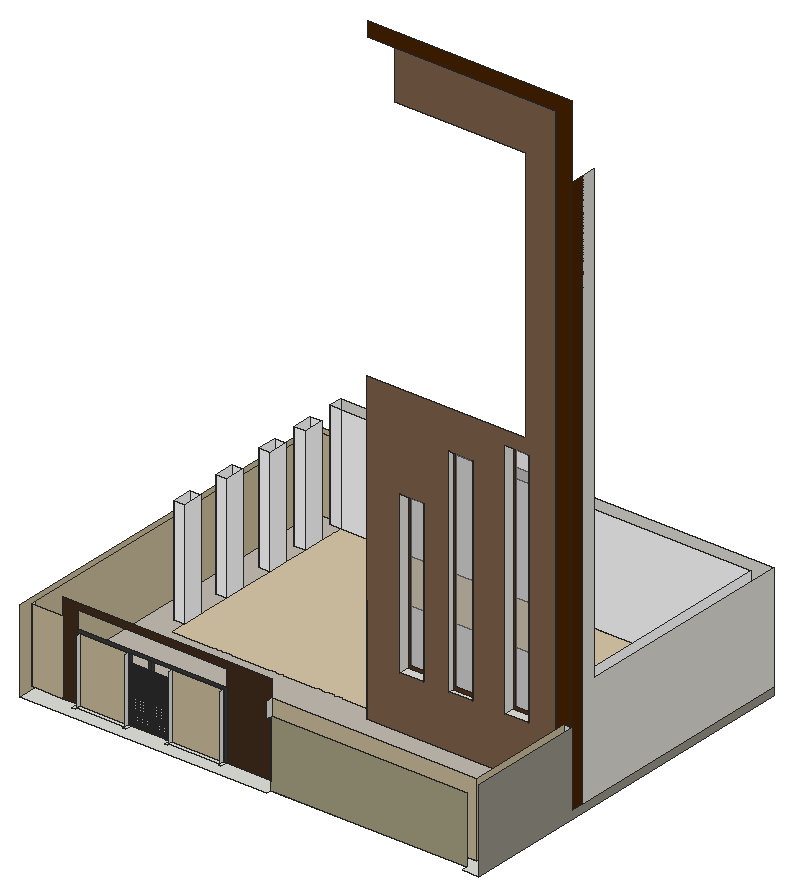
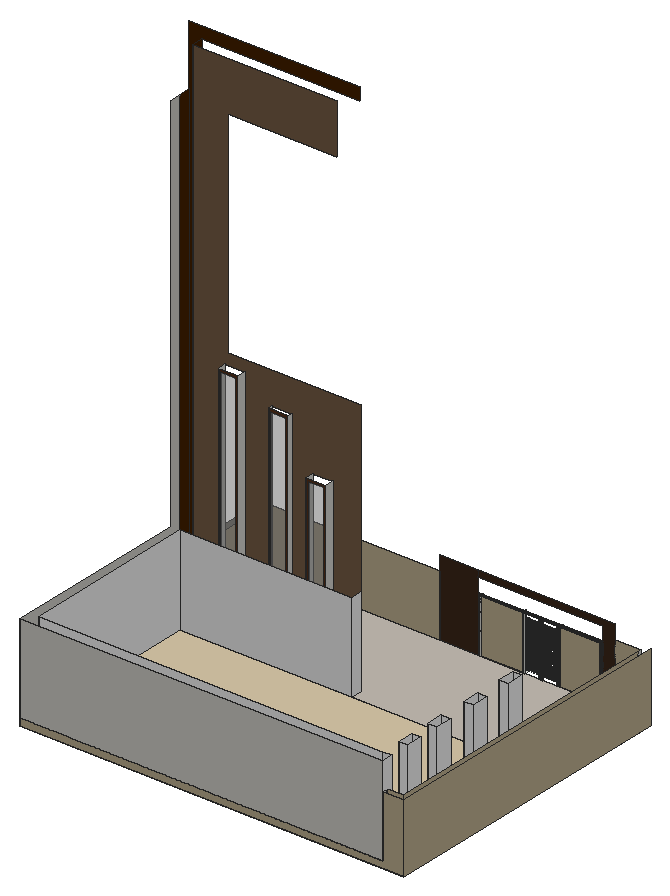
# SketchUp Ruby script. Lengths in inches.
U = 1.inch
M = Sketchup.active_model
def pt(a) = Geom::Point3d.new(a.map { |v| v * U })
def face(e, loops, mat)
  f = e.add_face(loops[0].map { |a| pt(a) })
  loops[1..].each { |l| e.add_face(l.map { |a| pt(a) }).erase! }
  f.material = f.back_material = mat if mat
  f
end
# faces: each face lists its corners as indices into pts; further lists are holes
def faces(e, pts, list, mat = nil) = list.each { |f| face(e, (f[0].is_a?(Array) ? f : [f]).map { |l| l.map { |i| pts[i] } }, mat) }
# xy, xz, yz: faces in a plane at the given z, y or x. An outline is a flat list of corners, or four numbers for a rectangle; further outlines are holes
def ring(l) = l.size == 4 ? [[l[0], l[1]], [l[2], l[1]], [l[2], l[3]], [l[0], l[3]]] : l.each_slice(2).to_a
def flat(e, list, mat, &to3) = list.each { |f| face(e, (f[0].is_a?(Array) ? f : [f]).map { |l| ring(l).map { |u, v| to3.(u, v) } }, mat) }
def xy(e, z, list, mat = nil) = flat(e, list, mat) { |x, y| [x, y, z] }
def xz(e, y, list, mat = nil) = flat(e, list, mat) { |x, z| [x, y, z] }
def yz(e, x, list, mat = nil) = flat(e, list, mat) { |y, z| [x, y, z] }
def lines(e, pts, list) = list.each { |a, b| e.add_line(pt(pts[a]), pt(pts[b])) }
# prism: a flat outline (further loops are holes) pulled along v
def prism(e, loops, v, mat = nil)
  f = face(e, loops, mat); d = Geom::Vector3d.new(v.map { |x| x * U })
  f.pushpull(f.normal.samedirection?(d) ? d.length : -d.length)
end
def box(e, o, s, mat = nil) = prism(e, [[o, [o[0] + s[0], o[1], o[2]], [o[0] + s[0], o[1] + s[1], o[2]], [o[0], o[1] + s[1], o[2]]]], [0, 0, s[2]], mat)
def at(x, y, z, deg = 0) = Geom::Transformation.translation(pt([x, y, z])) * Geom::Transformation.rotation(ORIGIN, Z_AXIS, deg.degrees)
def axes(o, x, y, z) = Geom::Transformation.new([*x, 0, *y, 0, *z, 0, *pt(o).to_a, 1])
def part(name) = M.definitions.add(name)
# library, detail: a bought-in or finely detailed component or shape, given as its bounding box
def library(name, o, s) = part(name).tap { |d| box(d.entities, o, s) }
def detail(e, o, s) = box(e.add_group.entities, o, s)
def put(e, d, t, mat = nil) = e.add_instance(d, t).tap { |i| i.material = mat if mat }
def group(e, t, mat = nil) = e.add_group.tap { |g| g.transformation = t; g.material = mat if mat }.entities
root = M.entities
M.materials.add("[Carrera Marble]").color = [252, 252, 252]
M.materials.add("[Carrera Marble]1").color = [247, 247, 247]
M.materials.add("[Cladding Siding Tan]").color = [124, 97, 73]
M.materials.add("[Color C08]").color = [71, 35, 0]
M.materials.add("[Color M07]").color = [58, 58, 58]
M.materials.add("[Field Rectangle Tile]").color = [196, 189, 179]
M.materials.add("[Field Square Tile]").color = [217, 201, 169]
M.materials.add("[Formica Graystone]1").color = [149, 146, 135]
M.materials.add("[Formica Speckled Grey]").color = [94, 105, 111]
M.materials.add("[Quartz Light Brown]").color = [199, 184, 152]
M.materials.add("[Sandstone]").color = [63, 43, 28]
M.materials.add("[Stone Coursed Rough]").color = [165, 160, 130]
M.materials.add("[Terrazzo Tile Light]").color = [219, 217, 210]
M.materials.add("[Translucent Glass Gray]1").color = [163, 163, 163]
M.materials["[Translucent Glass Gray]1"].alpha = 0.5
M.materials.add("[Wood Cherry Original]").color = [91, 51, 25]
xy(root,0,[[71.32,279.21,71.32,742.77,649.65,742.77,649.65,279.21,628.99,279.21,628.99,285.9,381.67,285.9,381.67,279.21]])
xy(root,10.08,[[136.3,279.21,140.74,288.34],[201.14,279.21,204.61,288.34],[253.76,279.21,256.89,288.34],[321.11,279.21,324.42,288.34],[140.74,281.7,201.14,286.88],
  [256.89,281.7,321.11,286.72],[256.89,286.72,321.11,288.34],[630.01,424.96,630.01,442.77,635.51,460.01,635.51,725.53,104.01,725.53,104.01,742.77,649.65,742.77,649.65,424.96],[376.83,442.77,376.83,460.01,635.51,460.01,630.01,442.77],[104.01,479.96,118.15,505.27],
  [104.01,546.4,118.15,571.71],[104.01,614.47,118.15,639.78],[104.01,670,118.15,695.31]])
xy(root,10.08,[[140.74,286.88,201.14,288.34]],"[Color M07]")
xy(root,10.08,[[78.57,288.34,639.83,288.34,639.83,424.96,630.01,424.96,630.01,442.77,376.83,442.77,376.83,460.01,118.15,460.01,118.15,479.96,104.01,479.96,104.01,505.27,118.15,505.27,118.15,546.4,104.01,546.4,104.01,571.71,118.15,571.71,118.15,614.47,104.01,614.47,104.01,639.78,118.15,639.78,118.15,670,104.01,670,104.01,695.31,118.15,695.31,118.15,725.53,104.01,725.53,104.01,734.15,78.57,734.15]],"[Field Rectangle Tile]")
xy(root,10.08,[[118.15,460.01,635.51,725.53]],"[Field Square Tile]")
xy(root,76.96,[[419.27,442.77,449.02,455.21],[480.71,442.77,510.46,449.52],[551.08,442.77,580.83,455.77]])
xz(root,285.9,[[381.67,0,628.99,83.9375]],"[Stone Coursed Rough]")
xz(root,286.72,[[256.89,10.08,321.11,91.34]],"[Quartz Light Brown]")
xz(root,286.88,[[140.74,10.08,201.14,91.34]],"[Quartz Light Brown]")
xz(root,288.34,[[253.76,10.08,256.89,91.34]])
xz(root,288.34,[[136.3,10.08,136.3,94.91,319.42,94.91,319.42,91.34,140.74,91.34,140.74,10.08],[201.14,10.08,204.61,91.34],[225.67,10.08,229.25,91.34],[229.25,10.08,232.82,91.34],[321.11,10.08,321.11,91.34,319.42,91.34,319.42,94.91,324.42,94.91,324.42,10.08]],"[Color M07]")
xz(root,288.34,[[78.57,10.08,118.15,103.14],[381.67,10.08,639.83,103.14]],"[Quartz Light Brown]")
xz(root,288.34,[[118.15,10.08,118.15,124.77,324.42,124.77,324.42,116.23,136.3,116.23,136.3,10.08],[324.42,10.08,381.67,124.77]],"[Sandstone]")
xz(root,424.96,[[639.83,10.08,649.65,103.14]])
xz(root,424.96,[[630.01,10.08,639.83,10.08,639.83,103.14,649.65,103.14,649.65,812.1,392.48,812.1,392.48,793.89,630.01,793.89]],"[Color C08]")
xz(root,442.77,[[[376.83,10.08,630.01,10.08,630.01,793.89,412.79,793.89,412.79,719.42,577.15,719.42,577.15,397.48,376.83,397.48],[551.08,76.96,580.83,380.34],[480.71,76.96,510.46,348.79],[419.27,76.96,449.02,278.96]]],"[Cladding Siding Tan]")
xz(root,449.52,[[484.53,80.79,506.63,344.96]],"[Translucent Glass Gray]1")
xz(root,449.52,[[[480.71,76.96,510.46,348.79],[484.53,80.79,506.63,344.96]]],"[Wood Cherry Original]")
xz(root,455.21,[[423.09,80.79,445.19,275.13]],"[Translucent Glass Gray]1")
xz(root,455.21,[[[419.27,76.96,449.02,278.96],[423.09,80.79,445.19,275.13]]],"[Wood Cherry Original]")
xz(root,455.77,[[554.91,80.79,577,376.52]],"[Translucent Glass Gray]1")
xz(root,455.77,[[[551.08,76.96,580.83,380.34],[554.91,80.79,577,376.52]]],"[Wood Cherry Original]")
xz(root,460.01,[[376.83,10.08,635.51,144.48]],"[Carrera Marble]1")
xz(root,479.96,[[104.01,10.08,118.15,144.48]],"[Carrera Marble]")
xz(root,505.27,[[104.01,10.08,118.15,144.48]],"[Carrera Marble]")
xz(root,546.4,[[104.01,10.08,118.15,144.48]],"[Carrera Marble]")
xz(root,571.71,[[104.01,10.08,118.15,144.48]],"[Carrera Marble]")
xz(root,614.47,[[104.01,10.08,118.15,144.48]],"[Carrera Marble]")
xz(root,639.78,[[104.01,10.08,118.15,144.48]],"[Carrera Marble]")
xz(root,670,[[104.01,10.08,118.15,144.48]],"[Carrera Marble]")
xz(root,695.31,[[104.01,10.08,118.15,144.48]],"[Carrera Marble]")
xz(root,725.53,[[118.15,10.08,635.51,144.48]],"[Carrera Marble]")
xz(root,725.53,[[104.01,10.08,118.15,144.48]],"[Carrera Marble]1")
xz(root,734.15,[[78.57,10.08,104.01,103.14]],"[Quartz Light Brown]")
xz(root,742.77,[[71.32,0,71.32,103.14,104.01,103.14,104.01,10.08,649.65,10.08,649.65,0]],"[Quartz Light Brown]")
xz(root,742.77,[[104.01,10.08,649.65,144.48]],"[Terrazzo Tile Light]")
yz(root,71.32,[[279.21,0,742.77,103.14]],"[Quartz Light Brown]")
yz(root,78.57,[[288.34,10.08,293.84,103.14]])
yz(root,78.57,[[293.84,10.08,734.15,103.14]],"[Quartz Light Brown]")
yz(root,104.01,[[734.15,10.08,742.77,103.14]])
yz(root,104.01,[[479.96,10.08,505.27,144.48],[546.4,10.08,571.71,144.48],[614.47,10.08,639.78,144.48],[670,10.08,695.31,144.48],[725.53,10.08,725.53,144.48,742.77,144.48,742.77,103.14,734.15,103.14,734.15,10.08]],"[Carrera Marble]")
yz(root,118.15,[[479.96,10.08,505.27,144.48],[546.4,10.08,571.71,144.48],[614.47,10.08,639.78,144.48],[670,10.08,695.31,144.48]],"[Carrera Marble]")
yz(root,140.74,[[281.7,10.08,286.88,91.34]])
yz(root,140.74,[[286.88,10.08,288.34,91.34]],"[Color M07]")
yz(root,201.14,[[281.7,10.08,286.88,91.34],[286.88,10.08,288.34,91.34]])
yz(root,256.89,[[281.7,10.08,286.72,91.34]])
yz(root,256.89,[[286.72,10.08,288.34,91.34]],"[Color M07]")
yz(root,321.11,[[281.7,10.08,286.72,91.34],[286.72,10.08,288.34,91.34]])
yz(root,376.83,[[442.77,10.08,460.01,144.48]],"[Carrera Marble]")
yz(root,381.67,[[285.9,10.08,288.34,10.08,288.34,103.14,279.21,103.14,279.21,83.9375,285.9,83.9375]])
yz(root,419.27,[[442.77,76.96,455.21,278.96]])
yz(root,449.02,[[442.77,76.96,455.21,278.96]])
yz(root,480.71,[[442.77,76.96,449.52,348.79]])
yz(root,510.46,[[442.77,76.96,449.52,348.79]])
yz(root,551.08,[[442.77,76.96,455.77,380.34]])
yz(root,580.83,[[442.77,76.96,455.77,380.34]])
yz(root,630.01,[[424.96,10.08,442.77,793.89]],"[Color C08]")
yz(root,635.51,[[460.01,10.08,725.53,144.48]],"[Carrera Marble]")
yz(root,639.83,[[288.34,10.08,424.96,103.14]],"[Quartz Light Brown]")
yz(root,649.65,[[424.96,10.08,442.77,719.42]],"[Color C08]")
yz(root,649.65,[[279.21,0,742.77,0,742.77,10.08,424.96,10.08,424.96,103.14,279.21,103.14]],"[Formica Graystone]1")
yz(root,649.65,[[442.77,10.08,742.77,10.08,742.77,144.48,460.01,144.48,460.01,719.42,442.77,719.42]],"[Terrazzo Tile Light]")
p = [[204.61,283.9,12.47],[204.61,284.05,12.53],[253.76,284.05,12.53],[253.76,283.9,12.47],[204.61,284.18,12.63],[253.76,284.18,12.63],
  [204.61,284.28,12.76],[253.76,284.28,12.76],[204.61,284.34,12.91],[253.76,284.34,12.91],[204.61,284.37,13.07],[253.76,284.37,13.07],
  [204.61,284.34,13.23],[253.76,284.34,13.23],[204.61,284.28,13.38],[253.76,284.28,13.38],[204.61,284.18,13.51],[253.76,284.18,13.51],
  [204.61,284.05,13.61],[253.76,284.05,13.61],[204.61,283.9,13.68],[253.76,283.9,13.68],[204.61,283.9,15.78],[204.61,284.05,15.84],
  [253.76,284.05,15.84],[253.76,283.9,15.78],[204.61,284.18,15.94],[253.76,284.18,15.94],[204.61,284.28,16.07],[253.76,284.28,16.07],
  [204.61,284.34,16.22],[253.76,284.34,16.22],[204.61,284.37,16.38],[253.76,284.37,16.38],[204.61,284.34,16.55],[253.76,284.34,16.55],
  [204.61,284.28,16.7],[253.76,284.28,16.7],[204.61,284.18,16.83],[253.76,284.18,16.83],[204.61,284.05,16.93],[253.76,284.05,16.93],
  [204.61,283.9,16.99],[253.76,283.9,16.99],[204.61,283.9,19.09],[204.61,284.05,19.16],[253.76,284.05,19.16],[253.76,283.9,19.09],
  [204.61,284.18,19.25],[253.76,284.18,19.25],[204.61,284.28,19.38],[253.76,284.28,19.38],[204.61,284.34,19.54],[253.76,284.34,19.54],
  [204.61,284.37,19.7],[253.76,284.37,19.7],[204.61,284.34,19.86],[253.76,284.34,19.86],[204.61,284.28,20.01],[253.76,284.28,20.01],
  [204.61,284.18,20.14],[253.76,284.18,20.14],[204.61,284.05,20.24],[253.76,284.05,20.24],[204.61,283.9,20.3],[253.76,283.9,20.3],
  [204.61,283.9,22.41],[204.61,284.05,22.47],[253.76,284.05,22.47],[253.76,283.9,22.41],[204.61,284.18,22.57],[253.76,284.18,22.57],
  [204.61,284.28,22.7],[253.76,284.28,22.7],[204.61,284.34,22.85],[253.76,284.34,22.85],[204.61,284.37,23.01],[253.76,284.37,23.01],
  [204.61,284.34,23.17],[253.76,284.34,23.17],[204.61,284.28,23.32],[253.76,284.28,23.32],[204.61,284.18,23.45],[253.76,284.18,23.45],
  [204.61,284.05,23.55],[253.76,284.05,23.55],[204.61,283.9,23.61],[253.76,283.9,23.61],[204.61,283.9,25.72],[204.61,284.05,25.78],
  [253.76,284.05,25.78],[253.76,283.9,25.72],[204.61,284.18,25.88],[253.76,284.18,25.88],[204.61,284.28,26.01],[253.76,284.28,26.01],
  [204.61,284.34,26.16],[253.76,284.34,26.16],[204.61,284.37,26.32],[253.76,284.37,26.32],[204.61,284.34,26.48],[253.76,284.34,26.48],
  [204.61,284.28,26.63],[253.76,284.28,26.63],[204.61,284.18,26.76],[253.76,284.18,26.76],[204.61,284.05,26.86],[253.76,284.05,26.86],
  [204.61,283.9,26.93],[253.76,283.9,26.93],[204.61,283.9,29.03],[204.61,284.05,29.09],[253.76,284.05,29.09],[253.76,283.9,29.03],
  [204.61,284.18,29.19],[253.76,284.18,29.19],[204.61,284.28,29.32],[253.76,284.28,29.32],[204.61,284.34,29.47],[253.76,284.34,29.47],
  [204.61,284.37,29.63],[253.76,284.37,29.63],[204.61,284.34,29.8],[253.76,284.34,29.8],[204.61,284.28,29.95],[253.76,284.28,29.95],
  [204.61,284.18,30.08],[253.76,284.18,30.08],[204.61,284.05,30.18],[253.76,284.05,30.18],[204.61,283.9,30.24],[253.76,283.9,30.24],
  [204.61,283.74,32.32],[204.61,283.9,32.34],[253.76,283.9,32.34],[253.76,283.74,32.32],[204.61,284.05,32.41],[253.76,284.05,32.41],
  [204.61,284.18,32.5],[253.76,284.18,32.5],[204.61,284.28,32.63],[253.76,284.28,32.63],[204.61,284.34,32.79],[253.76,284.34,32.79],
  [204.61,284.37,32.95],[253.76,284.37,32.95],[204.61,284.34,33.11],[253.76,284.34,33.11],[204.61,284.28,33.26],[253.76,284.28,33.26],
  [204.61,284.18,33.39],[253.76,284.18,33.39],[204.61,284.05,33.49],[253.76,284.05,33.49],[204.61,283.9,33.55],[253.76,283.9,33.55],
  [204.61,283.74,33.57],[253.76,283.74,33.57],[204.61,283.74,35.63],[204.61,283.9,35.66],[253.76,283.9,35.66],[253.76,283.74,35.63],
  [204.61,284.05,35.72],[253.76,284.05,35.72],[204.61,284.18,35.82],[253.76,284.18,35.82],[204.61,284.28,35.95],[253.76,284.28,35.95],
  [204.61,284.34,36.1],[253.76,284.34,36.1],[204.61,284.37,36.26],[253.76,284.37,36.26],[204.61,284.34,36.42],[253.76,284.34,36.42],
  [204.61,284.28,36.57],[253.76,284.28,36.57],[204.61,284.18,36.7],[253.76,284.18,36.7],[204.61,284.05,36.8],[253.76,284.05,36.8],
  [204.61,283.9,36.86],[253.76,283.9,36.86],[204.61,283.74,36.88],[253.76,283.74,36.88],[204.61,283.74,38.95],[204.61,283.9,38.97],
  [253.76,283.9,38.97],[253.76,283.74,38.95],[204.61,284.05,39.03],[253.76,284.05,39.03],[204.61,284.18,39.13],[253.76,284.18,39.13],
  [204.61,284.28,39.26],[253.76,284.28,39.26],[204.61,284.34,39.41],[253.76,284.34,39.41],[204.61,284.37,39.57],[253.76,284.37,39.57],
  [204.61,284.34,39.73],[253.76,284.34,39.73],[204.61,284.28,39.88],[253.76,284.28,39.88],[204.61,284.18,40.01],[253.76,284.18,40.01],
  [204.61,284.05,40.11],[253.76,284.05,40.11],[204.61,283.9,40.18],[253.76,283.9,40.18],[204.61,283.74,40.2],[253.76,283.74,40.2],
  [204.61,283.74,42.26],[204.61,283.9,42.28],[253.76,283.9,42.28],[253.76,283.74,42.26],[204.61,284.05,42.34],[253.76,284.05,42.34],
  [204.61,284.18,42.44],[253.76,284.18,42.44],[204.61,284.28,42.57],[253.76,284.28,42.57],[204.61,284.34,42.72],[253.76,284.34,42.72],
  [204.61,284.37,42.88],[253.76,284.37,42.88],[204.61,284.34,43.05],[253.76,284.34,43.05],[204.61,284.28,43.2],[253.76,284.28,43.2],
  [204.61,284.18,43.33],[253.76,284.18,43.33],[204.61,284.05,43.43],[253.76,284.05,43.43],[204.61,283.9,43.49],[253.76,283.9,43.49],
  [204.61,283.74,43.51],[253.76,283.74,43.51],[204.61,283.74,45.57],[204.61,283.9,45.59],[253.76,283.9,45.59],[253.76,283.74,45.57],
  [204.61,284.05,45.66],[253.76,284.05,45.66],[204.61,284.18,45.75],[253.76,284.18,45.75],[204.61,284.28,45.88],[253.76,284.28,45.88],
  [204.61,284.34,46.04],[253.76,284.34,46.04],[204.61,284.37,46.2],[253.76,284.37,46.2],[204.61,284.34,46.36],[253.76,284.34,46.36],
  [204.61,284.28,46.51],[253.76,284.28,46.51],[204.61,284.18,46.64],[253.76,284.18,46.64],[204.61,284.05,46.74],[253.76,284.05,46.74],
  [204.61,283.9,46.8],[253.76,283.9,46.8],[204.61,283.74,46.82],[253.76,283.74,46.82],[204.61,283.74,48.38],[204.61,283.9,48.41],
  [253.76,283.9,48.41],[253.76,283.74,48.38],[204.61,284.05,48.47],[253.76,284.05,48.47],[204.61,284.18,48.57],[253.76,284.18,48.57],
  [204.61,284.28,48.7],[253.76,284.28,48.7],[204.61,284.34,48.85],[253.76,284.34,48.85],[204.61,284.37,49.01],[253.76,284.37,49.01],
  [204.61,284.34,49.17],[253.76,284.34,49.17],[204.61,284.28,49.32],[253.76,284.28,49.32],[204.61,284.18,49.45],[253.76,284.18,49.45],
  [204.61,284.05,49.55],[253.76,284.05,49.55],[204.61,283.9,49.61],[204.61,283.74,49.63],[253.76,283.74,49.63],[253.76,283.9,49.61],
  [204.61,283.74,51.2],[204.61,283.9,51.22],[253.76,283.9,51.22],[253.76,283.74,51.2],[204.61,284.05,51.28],[253.76,284.05,51.28],
  [204.61,284.18,51.38],[253.76,284.18,51.38],[204.61,284.28,51.51],[253.76,284.28,51.51],[204.61,284.34,51.66],[253.76,284.34,51.66],
  [204.61,284.37,51.82],[253.76,284.37,51.82],[204.61,284.34,51.98],[253.76,284.34,51.98],[204.61,284.28,52.13],[253.76,284.28,52.13],
  [204.61,284.18,52.26],[253.76,284.18,52.26],[204.61,284.05,52.36],[253.76,284.05,52.36],[204.61,283.9,52.43],[204.61,283.74,52.45],
  [253.76,283.74,52.45],[253.76,283.9,52.43],[204.61,283.74,54.01],[204.61,283.9,54.03],[253.76,283.9,54.03],[253.76,283.74,54.01],
  [204.61,284.05,54.09],[253.76,284.05,54.09],[204.61,284.18,54.19],[253.76,284.18,54.19],[204.61,284.28,54.32],[253.76,284.28,54.32],
  [204.61,284.34,54.47],[253.76,284.34,54.47],[204.61,284.37,54.63],[253.76,284.37,54.63],[204.61,284.34,54.8],[253.76,284.34,54.8],
  [204.61,284.28,54.95],[253.76,284.28,54.95],[204.61,284.18,55.08],[253.76,284.18,55.08],[204.61,284.05,55.18],[253.76,284.05,55.18],
  [204.61,283.9,55.24],[204.61,283.74,55.26],[253.76,283.74,55.26],[253.76,283.9,55.24],[204.61,283.74,56.82],[204.61,283.9,56.84],
  [253.76,283.9,56.84],[253.76,283.74,56.82],[204.61,284.05,56.91],[253.76,284.05,56.91],[204.61,284.18,57],[253.76,284.18,57],
  [204.61,284.28,57.13],[253.76,284.28,57.13],[204.61,284.34,57.29],[253.76,284.34,57.29],[204.61,284.37,57.45],[253.76,284.37,57.45],
  [204.61,284.34,57.61],[253.76,284.34,57.61],[204.61,284.28,57.76],[253.76,284.28,57.76],[204.61,284.18,57.89],[253.76,284.18,57.89],
  [204.61,284.05,57.99],[253.76,284.05,57.99],[204.61,283.9,58.05],[253.76,283.9,58.05],[204.61,283.74,58.07],[253.76,283.74,58.07],
  [204.61,283.74,59.63],[204.61,283.9,59.66],[253.76,283.9,59.66],[253.76,283.74,59.63],[204.61,284.05,59.72],[253.76,284.05,59.72],
  [204.61,284.18,59.82],[253.76,284.18,59.82],[204.61,284.28,59.95],[253.76,284.28,59.95],[204.61,284.34,60.1],[253.76,284.34,60.1],
  [204.61,284.37,60.26],[253.76,284.37,60.26],[204.61,284.34,60.42],[253.76,284.34,60.42],[204.61,284.28,60.57],[253.76,284.28,60.57],
  [204.61,284.18,60.7],[253.76,284.18,60.7],[204.61,284.05,60.8],[253.76,284.05,60.8],[204.61,283.9,60.86],[253.76,283.9,60.86],
  [204.61,283.74,60.88],[253.76,283.74,60.88],[204.61,283.74,62.45],[204.61,283.9,62.47],[253.76,283.9,62.47],[253.76,283.74,62.45],
  [204.61,284.05,62.53],[253.76,284.05,62.53],[204.61,284.18,62.63],[253.76,284.18,62.63],[204.61,284.28,62.76],[253.76,284.28,62.76],
  [204.61,284.34,62.91],[253.76,284.34,62.91],[204.61,284.37,63.07],[253.76,284.37,63.07],[204.61,284.34,63.23],[253.76,284.34,63.23],
  [204.61,284.28,63.38],[253.76,284.28,63.38],[204.61,284.18,63.51],[253.76,284.18,63.51],[204.61,284.05,63.61],[253.76,284.05,63.61],
  [204.61,283.9,63.68],[253.76,283.9,63.68],[204.61,283.74,63.7],[253.76,283.74,63.7],[204.61,283.74,65.26],[204.61,283.9,65.28],
  [253.76,283.9,65.28],[253.76,283.74,65.26],[204.61,284.05,65.34],[253.76,284.05,65.34],[204.61,284.18,65.44],[253.76,284.18,65.44],
  [204.61,284.28,65.57],[253.76,284.28,65.57],[204.61,284.34,65.72],[253.76,284.34,65.72],[204.61,284.37,65.88],[253.76,284.37,65.88],
  [204.61,284.34,66.05],[253.76,284.34,66.05],[204.61,284.28,66.2],[253.76,284.28,66.2],[204.61,284.18,66.33],[253.76,284.18,66.33],
  [204.61,284.05,66.43],[253.76,284.05,66.43],[204.61,283.9,66.49],[253.76,283.9,66.49],[204.61,283.74,66.51],[253.76,283.74,66.51],
  [204.61,283.74,68.07],[204.61,283.9,68.09],[253.76,283.9,68.09],[253.76,283.74,68.07],[204.61,284.05,68.16],[253.76,284.05,68.16],
  [204.61,284.18,68.25],[253.76,284.18,68.25],[204.61,284.28,68.38],[253.76,284.28,68.38],[204.61,284.34,68.54],[253.76,284.34,68.54],
  [204.61,284.37,68.7],[253.76,284.37,68.7],[204.61,284.34,68.86],[253.76,284.34,68.86],[204.61,284.28,69.01],[253.76,284.28,69.01],
  [204.61,284.18,69.14],[253.76,284.18,69.14],[204.61,284.05,69.24],[253.76,284.05,69.24],[204.61,283.9,69.3],[253.76,283.9,69.3],
  [204.61,283.74,69.32],[253.76,283.74,69.32],[204.61,283.74,70.88],[204.61,283.9,70.91],[253.76,283.9,70.91],[253.76,283.74,70.88],
  [204.61,284.05,70.97],[253.76,284.05,70.97],[204.61,284.18,71.07],[253.76,284.18,71.07],[204.61,284.28,71.2],[253.76,284.28,71.2],
  [204.61,284.34,71.35],[253.76,284.34,71.35],[204.61,284.37,71.51],[253.76,284.37,71.51],[204.61,284.34,71.67],[253.76,284.34,71.67],
  [204.61,284.28,71.82],[253.76,284.28,71.82],[204.61,284.18,71.95],[253.76,284.18,71.95],[204.61,284.05,72.05],[253.76,284.05,72.05],
  [204.61,283.9,72.11],[204.61,283.74,72.13],[253.76,283.74,72.13],[253.76,283.9,72.11],[204.61,283.74,73.7],[204.61,283.9,73.72],
  [253.76,283.9,73.72],[253.76,283.74,73.7],[204.61,284.05,73.78],[253.76,284.05,73.78],[204.61,284.18,73.88],[253.76,284.18,73.88],
  [204.61,284.28,74.01],[253.76,284.28,74.01],[204.61,284.34,74.16],[253.76,284.34,74.16],[204.61,284.37,74.32],[253.76,284.37,74.32],
  [204.61,284.34,74.48],[253.76,284.34,74.48],[204.61,284.28,74.63],[253.76,284.28,74.63],[204.61,284.18,74.76],[253.76,284.18,74.76],
  [204.61,284.05,74.86],[253.76,284.05,74.86],[204.61,283.9,74.93],[204.61,283.74,74.95],[253.76,283.74,74.95],[253.76,283.9,74.93],
  [204.61,283.74,76.51],[204.61,283.9,76.53],[253.76,283.9,76.53],[253.76,283.74,76.51],[204.61,284.05,76.59],[253.76,284.05,76.59],
  [204.61,284.18,76.69],[253.76,284.18,76.69],[204.61,284.28,76.82],[253.76,284.28,76.82],[204.61,284.34,76.97],[253.76,284.34,76.97],
  [204.61,284.37,77.13],[253.76,284.37,77.13],[204.61,284.34,77.3],[253.76,284.34,77.3],[204.61,284.28,77.45],[253.76,284.28,77.45],
  [204.61,284.18,77.58],[253.76,284.18,77.58],[204.61,284.05,77.68],[253.76,284.05,77.68],[204.61,283.9,77.74],[204.61,283.74,77.76],
  [253.76,283.74,77.76],[253.76,283.9,77.74],[204.61,283.74,79.32],[204.61,283.9,79.34],[253.76,283.9,79.34],[253.76,283.74,79.32],
  [204.61,284.05,79.41],[253.76,284.05,79.41],[204.61,284.18,79.5],[253.76,284.18,79.5],[204.61,284.28,79.63],[253.76,284.28,79.63],
  [204.61,284.34,79.79],[253.76,284.34,79.79],[204.61,284.37,79.95],[253.76,284.37,79.95],[204.61,284.34,80.11],[253.76,284.34,80.11],
  [204.61,284.28,80.26],[253.76,284.28,80.26],[204.61,284.18,80.39],[253.76,284.18,80.39],[204.61,284.05,80.49],[253.76,284.05,80.49],
  [204.61,283.9,80.55],[253.76,283.9,80.55],[204.61,283.74,80.57],[253.76,283.74,80.57],[204.61,283.74,82.13],[204.61,283.9,82.16],
  [253.76,283.9,82.16],[253.76,283.74,82.13],[204.61,284.05,82.22],[253.76,284.05,82.22],[204.61,284.18,82.32],[253.76,284.18,82.32],
  [204.61,284.28,82.45],[253.76,284.28,82.45],[204.61,284.34,82.6],[253.76,284.34,82.6],[204.61,284.37,82.76],[253.76,284.37,82.76],
  [204.61,284.34,82.92],[253.76,284.34,82.92],[204.61,284.28,83.07],[253.76,284.28,83.07],[204.61,284.18,83.2],[253.76,284.18,83.2],
  [204.61,284.05,83.3],[253.76,284.05,83.3],[204.61,283.9,83.36],[253.76,283.9,83.36],[204.61,283.74,83.38],[253.76,283.74,83.38]]
faces(root,p,[[0,1,2,3],[1,4,5,2],[4,6,7,5],[6,8,9,7],[8,10,11,9],[10,12,13,11],[12,14,15,13],[14,16,17,15],
  [16,18,19,17],[18,20,21,19],[22,23,24,25],[23,26,27,24],[26,28,29,27],[28,30,31,29],[30,32,33,31],[32,34,35,33],
  [34,36,37,35],[36,38,39,37],[38,40,41,39],[40,42,43,41],[44,45,46,47],[45,48,49,46],[48,50,51,49],[50,52,53,51],
  [52,54,55,53],[54,56,57,55],[56,58,59,57],[58,60,61,59],[60,62,63,61],[62,64,65,63],[66,67,68,69],[67,70,71,68],
  [70,72,73,71],[72,74,75,73],[74,76,77,75],[76,78,79,77],[78,80,81,79],[80,82,83,81],[82,84,85,83],[84,86,87,85],
  [88,89,90,91],[89,92,93,90],[92,94,95,93],[94,96,97,95],[96,98,99,97],[98,100,101,99],[100,102,103,101],[102,104,105,103],
  [104,106,107,105],[106,108,109,107],[110,111,112,113],[111,114,115,112],[114,116,117,115],[116,118,119,117],[118,120,121,119],[120,122,123,121],
  [122,124,125,123],[124,126,127,125],[126,128,129,127],[128,130,131,129],[132,133,134,135],[133,136,137,134],[136,138,139,137],[138,140,141,139],
  [140,142,143,141],[142,144,145,143],[144,146,147,145],[146,148,149,147],[148,150,151,149],[150,152,153,151],[152,154,155,153],[154,156,157,155],
  [158,159,160,161],[159,162,163,160],[162,164,165,163],[164,166,167,165],[166,168,169,167],[168,170,171,169],[170,172,173,171],[172,174,175,173],
  [174,176,177,175],[176,178,179,177],[178,180,181,179],[180,182,183,181],[184,185,186,187],[185,188,189,186],[188,190,191,189],[190,192,193,191],
  [192,194,195,193],[194,196,197,195],[196,198,199,197],[198,200,201,199],[200,202,203,201],[202,204,205,203],[204,206,207,205],[206,208,209,207],
  [210,211,212,213],[211,214,215,212],[214,216,217,215],[216,218,219,217],[218,220,221,219],[220,222,223,221],[222,224,225,223],[224,226,227,225],
  [226,228,229,227],[228,230,231,229],[230,232,233,231],[232,234,235,233],[236,237,238,239],[237,240,241,238],[240,242,243,241],[242,244,245,243],
  [244,246,247,245],[246,248,249,247],[248,250,251,249],[250,252,253,251],[252,254,255,253],[254,256,257,255],[256,258,259,257],[258,260,261,259],
  [262,263,264,265],[263,266,267,264],[266,268,269,267],[268,270,271,269],[270,272,273,271],[272,274,275,273],[274,276,277,275],[276,278,279,277],
  [278,280,281,279],[280,282,283,281],[284,285,286,287],[282,284,287,283],[288,289,290,291],[289,292,293,290],[292,294,295,293],[294,296,297,295],
  [296,298,299,297],[298,300,301,299],[300,302,303,301],[302,304,305,303],[304,306,307,305],[306,308,309,307],[310,311,312,313],[308,310,313,309],
  [314,315,316,317],[315,318,319,316],[318,320,321,319],[320,322,323,321],[322,324,325,323],[324,326,327,325],[326,328,329,327],[328,330,331,329],
  [330,332,333,331],[332,334,335,333],[336,337,338,339],[334,336,339,335],[340,341,342,343],[341,344,345,342],[344,346,347,345],[346,348,349,347],
  [348,350,351,349],[350,352,353,351],[352,354,355,353],[354,356,357,355],[356,358,359,357],[358,360,361,359],[360,362,363,361],[362,364,365,363],
  [366,367,368,369],[367,370,371,368],[370,372,373,371],[372,374,375,373],[374,376,377,375],[376,378,379,377],[378,380,381,379],[380,382,383,381],
  [382,384,385,383],[384,386,387,385],[386,388,389,387],[388,390,391,389],[392,393,394,395],[393,396,397,394],[396,398,399,397],[398,400,401,399],
  [400,402,403,401],[402,404,405,403],[404,406,407,405],[406,408,409,407],[408,410,411,409],[410,412,413,411],[412,414,415,413],[414,416,417,415],
  [418,419,420,421],[419,422,423,420],[422,424,425,423],[424,426,427,425],[426,428,429,427],[428,430,431,429],[430,432,433,431],[432,434,435,433],
  [434,436,437,435],[436,438,439,437],[438,440,441,439],[440,442,443,441],[444,445,446,447],[445,448,449,446],[448,450,451,449],[450,452,453,451],
  [452,454,455,453],[454,456,457,455],[456,458,459,457],[458,460,461,459],[460,462,463,461],[462,464,465,463],[464,466,467,465],[466,468,469,467],
  [470,471,472,473],[471,474,475,472],[474,476,477,475],[476,478,479,477],[478,480,481,479],[480,482,483,481],[482,484,485,483],[484,486,487,485],
  [486,488,489,487],[488,490,491,489],[492,493,494,495],[490,492,495,491],[496,497,498,499],[497,500,501,498],[500,502,503,501],[502,504,505,503],
  [504,506,507,505],[506,508,509,507],[508,510,511,509],[510,512,513,511],[512,514,515,513],[514,516,517,515],[518,519,520,521],[516,518,521,517],
  [522,523,524,525],[523,526,527,524],[526,528,529,527],[528,530,531,529],[530,532,533,531],[532,534,535,533],[534,536,537,535],[536,538,539,537],
  [538,540,541,539],[540,542,543,541],[544,545,546,547],[542,544,547,543],[548,549,550,551],[549,552,553,550],[552,554,555,553],[554,556,557,555],
  [556,558,559,557],[558,560,561,559],[560,562,563,561],[562,564,565,563],[564,566,567,565],[566,568,569,567],[568,570,571,569],[570,572,573,571],
  [574,575,576,577],[575,578,579,576],[578,580,581,579],[580,582,583,581],[582,584,585,583],[584,586,587,585],[586,588,589,587],[588,590,591,589],
  [590,592,593,591],[592,594,595,593],[594,596,597,595],[596,598,599,597]],"[Formica Speckled Grey]")
